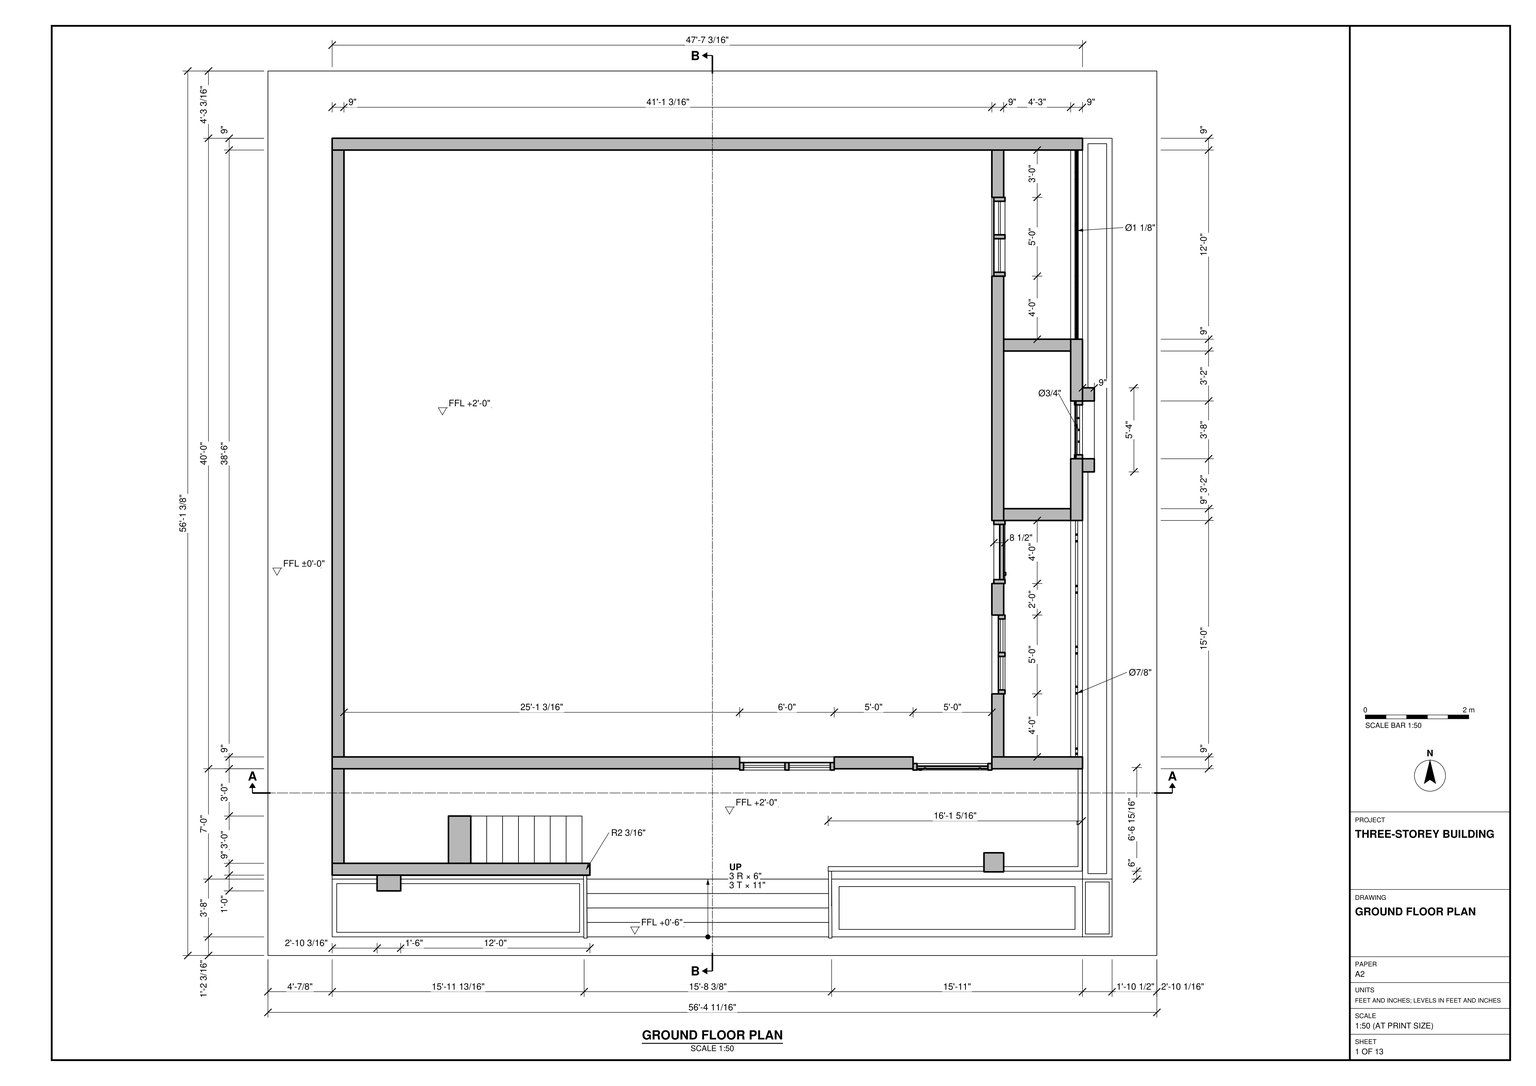
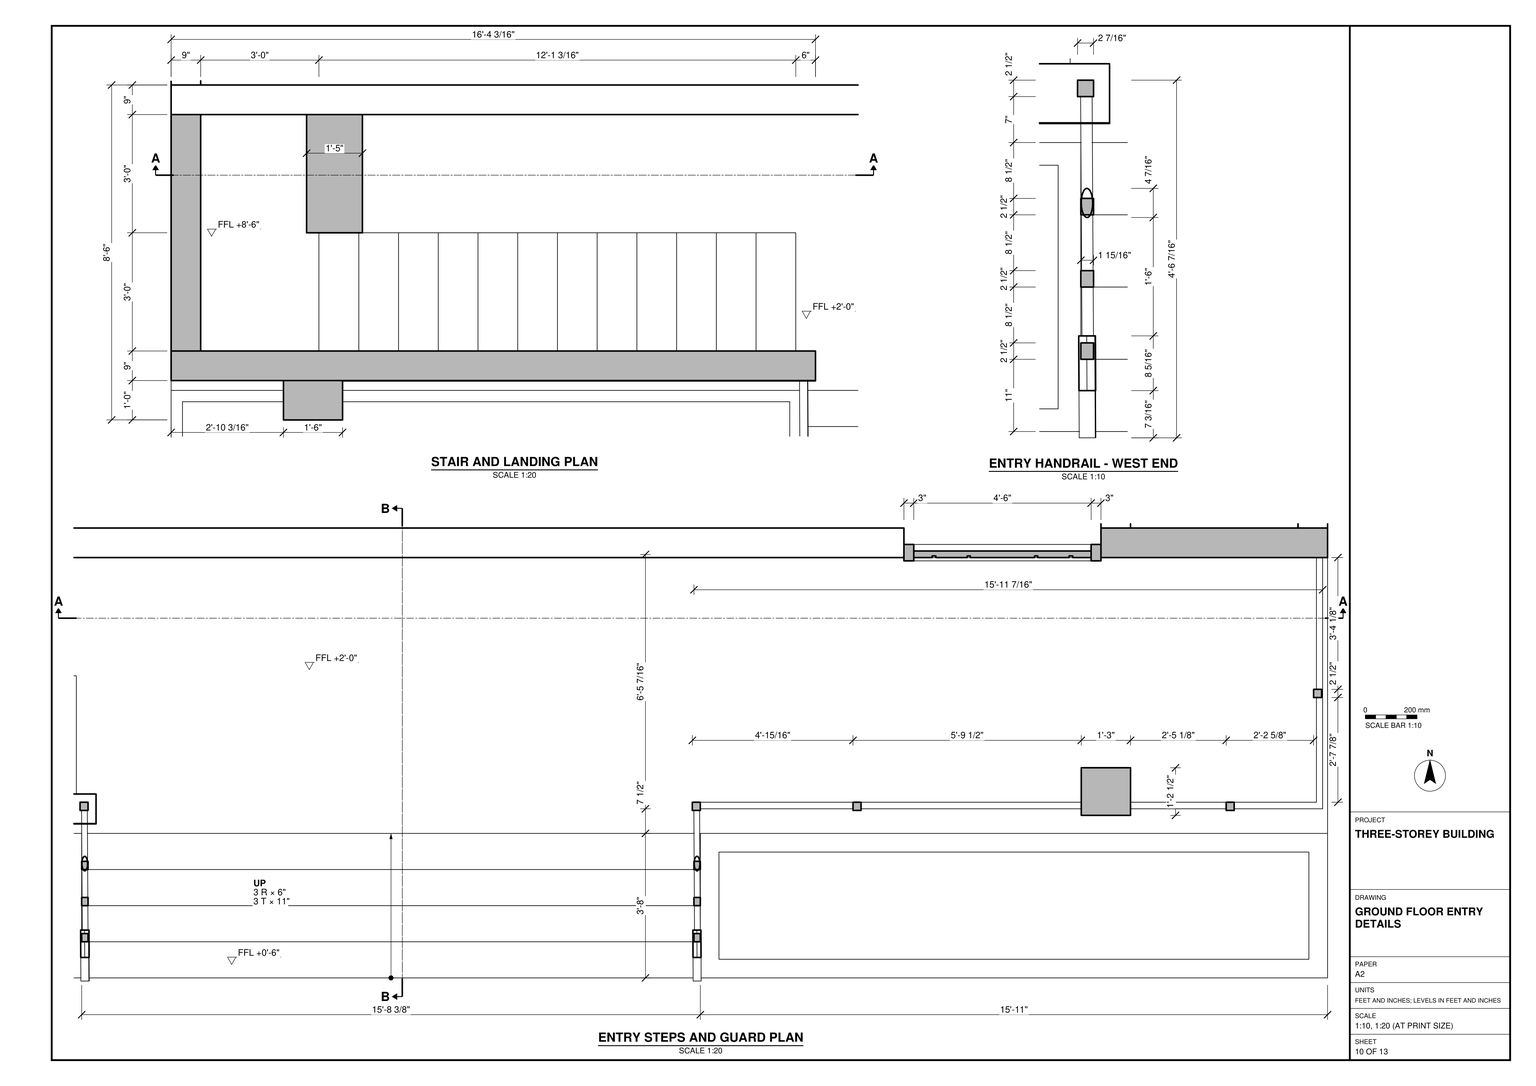
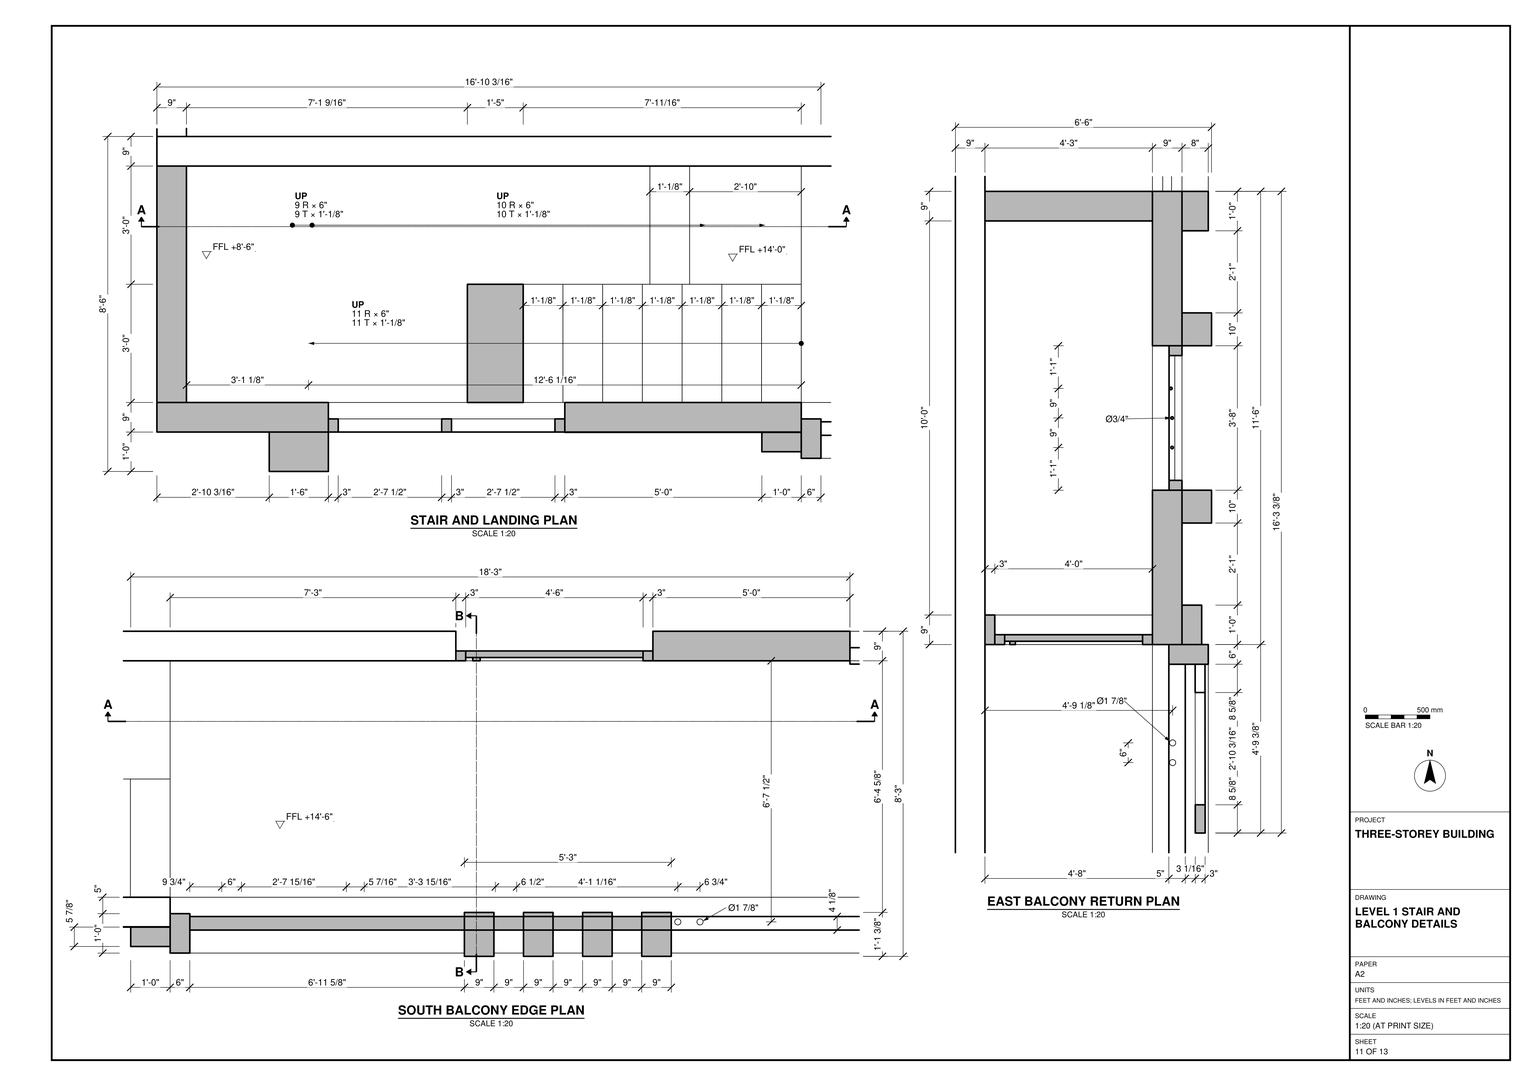
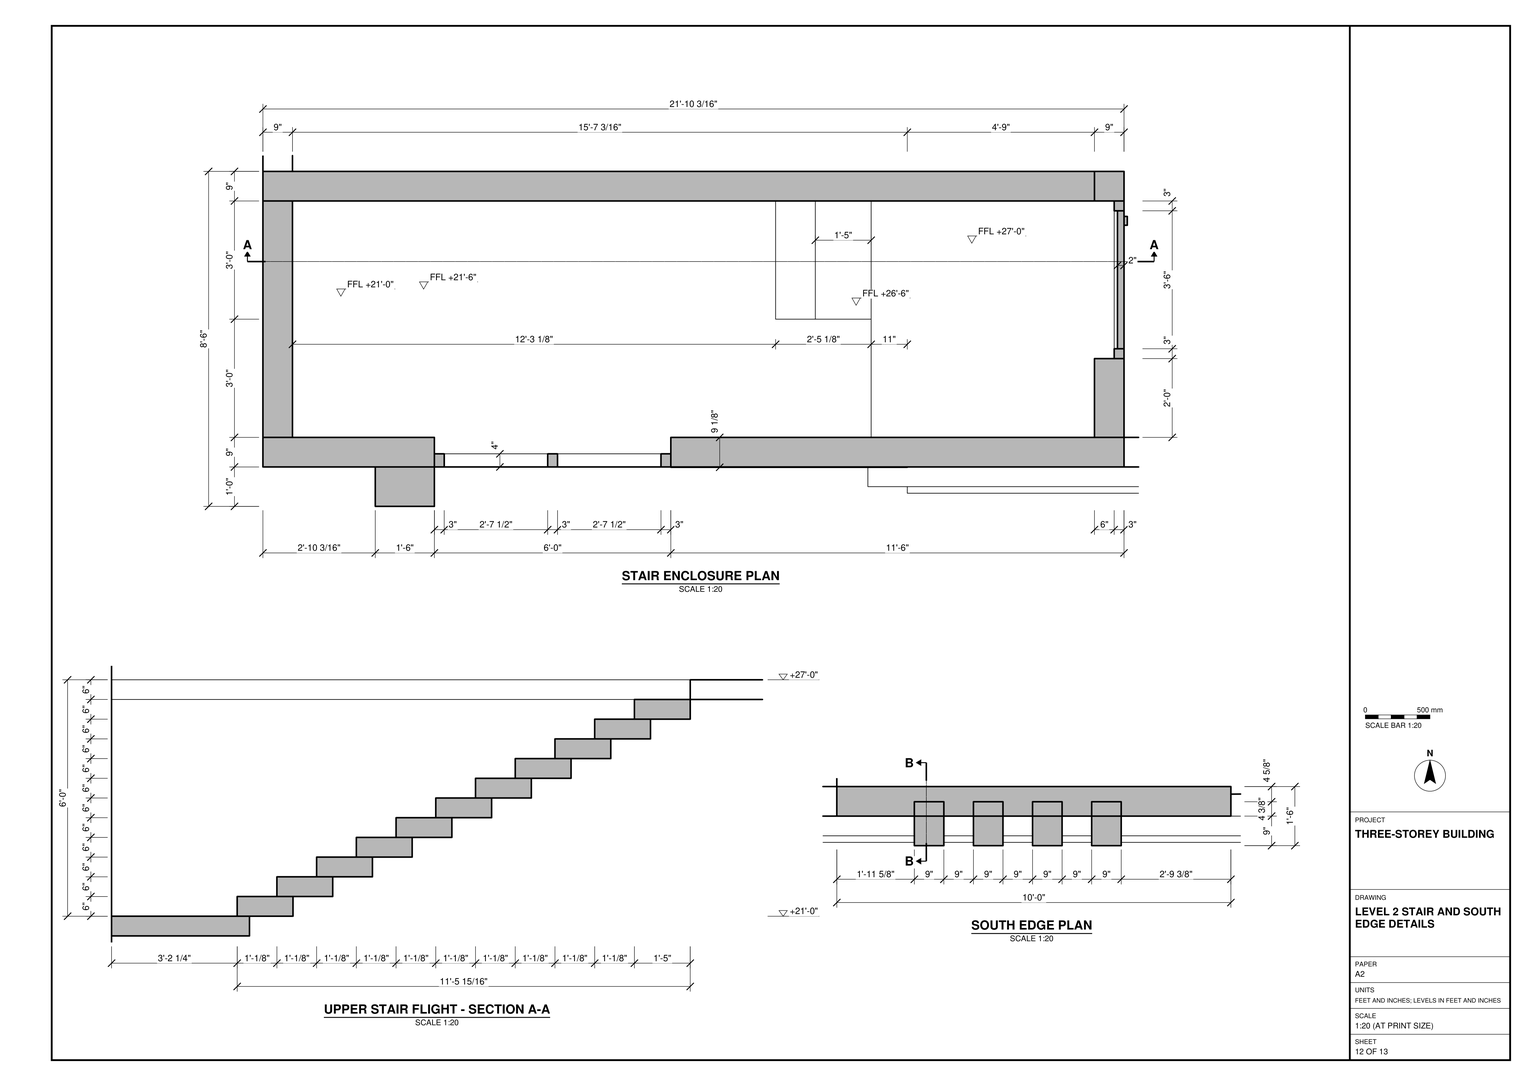
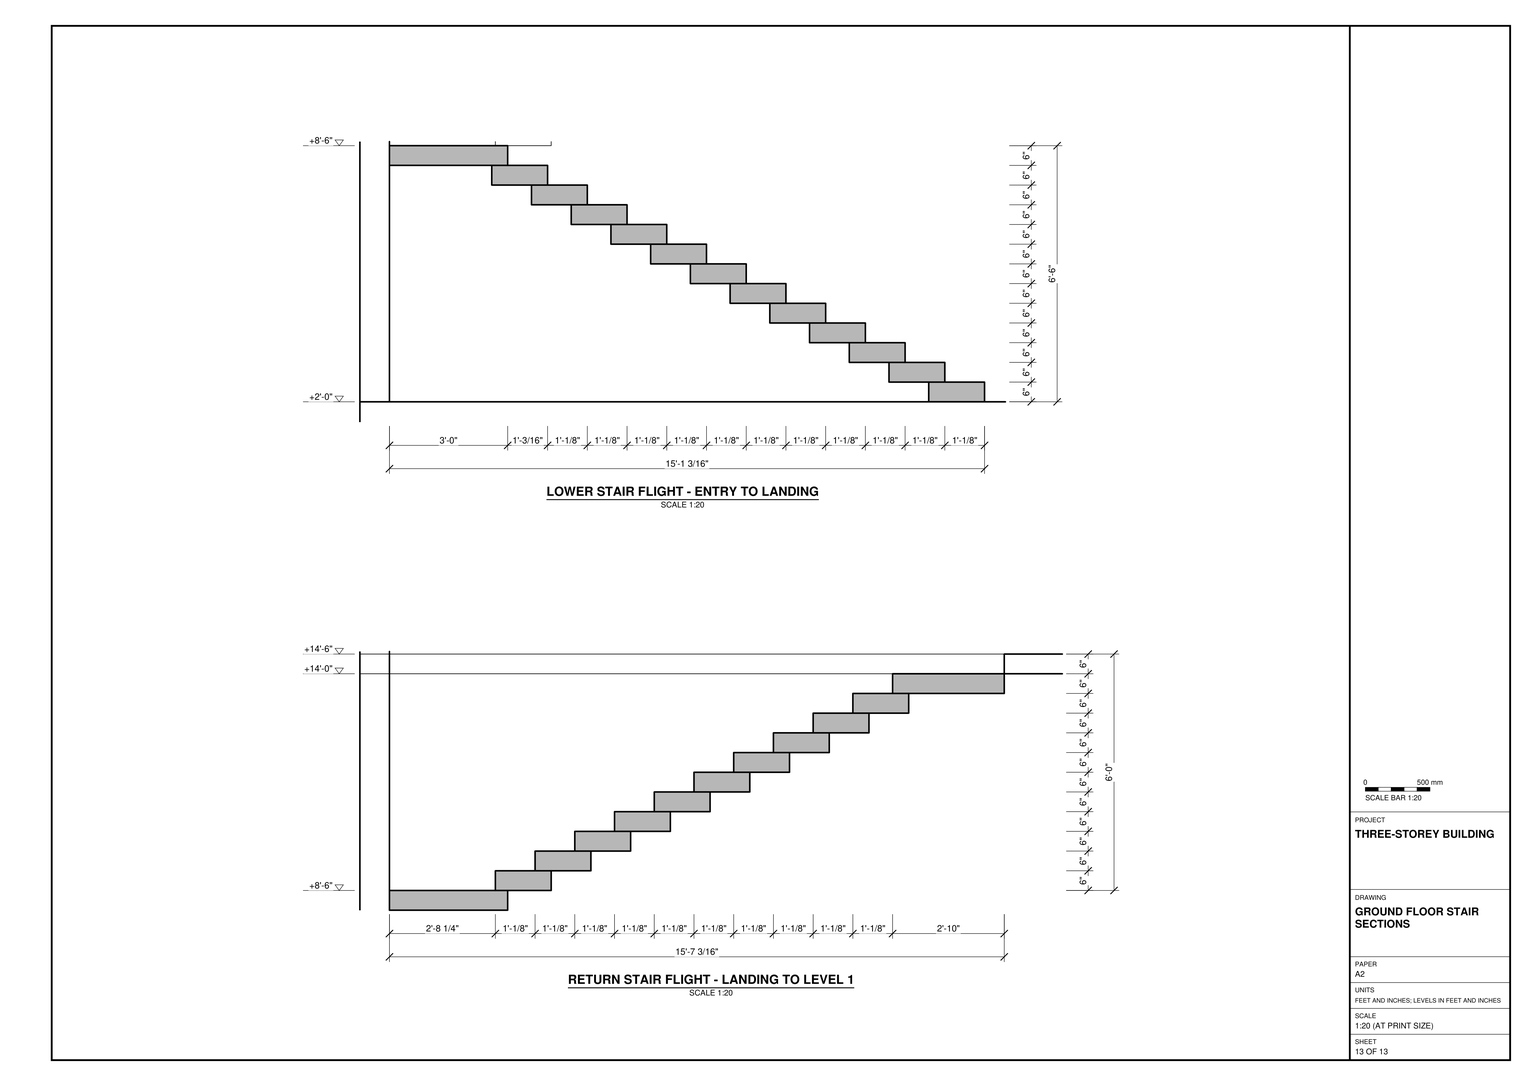
Build the three-storey building in SketchUp using task_files/diagram_01.pdf. Work in feet and inches. Orient the south entrance as shown on the plan. The overall model measures 56'-4 11/16" east to west, 56'-1 3/8" north to south and 43'-0" high. Use ±0'-0" as the ground datum and set the upper storey levels at +14'-6" and +27'-0". Distinguish the raised ground-floor surface at +2'-0" from the surrounding base.

Lay out the large open ground-floor space, the narrow bays along its east side and the entrance along its south side. Use the wall thicknesses shown, including the 9" walls, and place the door and window openings to match the plans. Model the broad entry steps and their handrails separately from the returning stair at the west end of the entrance. Align the stair flights, intermediate landings and slab openings so the stair connects the levels shown. Use the balcony details to shape the south edge and east return, including their guards. Complete the upper walls, floor slabs and roof to match the sheets.

Keep walls, slabs, roof and any furniture or built-in joinery shown as separate groups or components, and use components for repeated parts. Decor and loose items may be any suitable library components. Save one SketchUp model as output_files/three_storey_building_with_a_raised_entry_and_balconies.skp.

# SketchUp Ruby script. Lengths in inches.
U = 1.inch
M = Sketchup.active_model
def pt(a) = Geom::Point3d.new(a.map { |v| v * U })
def face(e, loops, mat)
  f = e.add_face(loops[0].map { |a| pt(a) })
  loops[1..].each { |l| e.add_face(l.map { |a| pt(a) }).erase! }
  f.material = f.back_material = mat if mat
  f
end
# faces: each face lists its corners as indices into pts; further lists are holes
def faces(e, pts, list, mat = nil) = list.each { |f| face(e, (f[0].is_a?(Array) ? f : [f]).map { |l| l.map { |i| pts[i] } }, mat) }
# xy, xz, yz: faces in a plane at the given z, y or x. An outline is a flat list of corners, or four numbers for a rectangle; further outlines are holes
def ring(l) = l.size == 4 ? [[l[0], l[1]], [l[2], l[1]], [l[2], l[3]], [l[0], l[3]]] : l.each_slice(2).to_a
def flat(e, list, mat, &to3) = list.each { |f| face(e, (f[0].is_a?(Array) ? f : [f]).map { |l| ring(l).map { |u, v| to3.(u, v) } }, mat) }
def xy(e, z, list, mat = nil) = flat(e, list, mat) { |x, y| [x, y, z] }
def xz(e, y, list, mat = nil) = flat(e, list, mat) { |x, z| [x, y, z] }
def yz(e, x, list, mat = nil) = flat(e, list, mat) { |y, z| [x, y, z] }
def lines(e, pts, list) = list.each { |a, b| e.add_line(pt(pts[a]), pt(pts[b])) }
# prism: a flat outline (further loops are holes) pulled along v
def prism(e, loops, v, mat = nil)
  f = face(e, loops, mat); d = Geom::Vector3d.new(v.map { |x| x * U })
  f.pushpull(f.normal.samedirection?(d) ? d.length : -d.length)
end
def box(e, o, s, mat = nil) = prism(e, [[o, [o[0] + s[0], o[1], o[2]], [o[0] + s[0], o[1] + s[1], o[2]], [o[0], o[1] + s[1], o[2]]]], [0, 0, s[2]], mat)
def at(x, y, z, deg = 0) = Geom::Transformation.translation(pt([x, y, z])) * Geom::Transformation.rotation(ORIGIN, Z_AXIS, deg.degrees)
def axes(o, x, y, z) = Geom::Transformation.new([*x, 0, *y, 0, *z, 0, *pt(o).to_a, 1])
def part(name) = M.definitions.add(name)
# library, detail: a bought-in or finely detailed component or shape, given as its bounding box
def library(name, o, s) = part(name).tap { |d| box(d.entities, o, s) }
def detail(e, o, s) = box(e.add_group.entities, o, s)
def put(e, d, t, mat = nil) = e.add_instance(d, t).tap { |i| i.material = mat if mat }
def group(e, t, mat = nil) = e.add_group.tap { |g| g.transformation = t; g.material = mat if mat }.entities
root = M.entities
M.materials.add("[Aluminum]").color = [179, 179, 179]
M.materials.add("[Color M01]").color = [226, 226, 226]
M.materials.add("[Color M02]").color = [198, 198, 198]
M.materials.add("[Color M03]").color = [170, 170, 170]
M.materials.add("[Color M06]").color = [86, 86, 86]
M.materials.add("[Color M09]").color = [0, 0, 0]
M.materials.add("[Grass Dark Green]").color = [106, 157, 55]
M.materials.add("[Metal Aluminum Anodized]").color = [202, 209, 219]
M.materials.add("[Metal Silver]").color = [234, 233, 238]
M.materials.add("[Translucent Glass Blue]").color = [100, 149, 237]
M.materials["[Translucent Glass Blue]"].alpha = 0.5
M.materials.add("[Translucent Glass Gray]").color = [128, 128, 128]
M.materials["[Translucent Glass Gray]"].alpha = 0.5
M.materials.add("[Wood Bamboo]").color = [177, 105, 43]
c1 = library("Group\#10",[0,0,0],[1.375,93,1.375])
c2 = library("Group\#22",[0,0,0],[2,54,2])
c3 = part("Group\#67")
box(c3.entities,[-6,0,0],[17,36,6])
c4 = part("Group\#17")
put(c4.entities,c3,at(102.77,0,18))
put(c4.entities,c3,at(139.05,0,0))
put(c4.entities,c3,at(30.19,0,54))
put(c4.entities,c3,at(78.58,0,30))
put(c4.entities,c3,at(42.29,0,48))
put(c4.entities,c3,at(18.1,0,60))
put(c4.entities,c3,at(90.67,0,24))
put(c4.entities,c3,at(126.96,0,6))
put(c4.entities,c3,at(66.48,0,36))
put(c4.entities,c3,at(54.38,0,42))
put(c4.entities,c3,at(114.86,0,12))
put(c4.entities,c3,at(6,0,66))
c5 = library("Group\#30",[0,0,0],[66,1.5,1.5])
c6 = library("Group\#33",[0,0,0],[54,2,102])
c7 = library("Group\#43",[0,0,0],[1,54,1])
c8 = library("Group\#16",[0,0,0],[1.625,38,69])
c9 = library("Group\#142",[0,0,0],[1.625,38,69])
c10 = library("Group\#51",[0,0,0],[66,2,2])
c11 = part("Group\#60")
box(c11.entities,[0,0,0],[4,2.91,144])
c12 = library("Group\#63",[0,0,0],[1.625,144,1.625])
c13 = library("Group\#64",[0,0,0],[0.75,0.75,30.1875])
c14 = part("Group\#72")
prism(c14.entities,[[[0,0,0],[0,3.125,0],[365,3.125,0],[365,264,0],[370,264,0],[370,0,0]]],[0,0,1.75])
c15 = library("Group\#73",[0,0,0],[1.875,1.875,35])
c16 = library("Group\#77",[0,0,0],[1.75,180,1.75])
c17 = library("Group\#78",[0,0,0],[0.875,0.875,22.1875])
c18 = library("Group\#80",[0,0,0],[2.625,144,2.625])
c19 = library("Group\#81",[0,0,0],[1.125,1.125,21.4375])
c20 = library("Group\#86",[0,0,0],[72,4,264])
c21 = part("Group\#118")
prism(c21.entities,[[[0,0,0],[0,5.25,0],[142.22,5.25,0],[142.22,83.66,0],[0,83.66,0],[0,88.35,0],[147.34,88.35,0],[147.34,0,0]]],[0,0,1.8125])
c22 = library("Group\#119",[0,0,0],[1.875,1.875,16.1875])
c23 = part("Group\#122")
prism(c23.entities,[[[0,0.5,0],[0,2.5,0],[189.55,2.5,0],[189.55,77.9375,0],[191.4375,77.9375,0],[191.4375,0.5,0]]],[0,0,3])
c24 = part("Group\#121")
box(c24.entities,[-0.5,0,0],[2.4375,2.5,36])
c25 = library("Group\#144",[0,0,0],[2.7,54.46,57])
c26 = library("Group\#130",[0,0,0],[2.8,54.46,57])
c27 = library("Group\#140",[0,0,0],[0.625,41,0.625])
c28 = library("Group\#141",[0,0,0],[0.875,41,0.875])
xz(root,61.08,[[240.23,64.88,242.67,67.88]])
xz(root,142.18,[[616.7,34,618.59,37],[616.7,42,618.59,45],[616.7,50,618.59,53],[616.7,58,618.59,61],[616.7,66,619.79,69]])
yz(root,560.09,[[65.68,42,67.68,45],[65.68,50,67.68,53],[65.68,58,67.68,61],[64.18,66,67.68,69]])
# 98 loose lines left out
g1 = group(root,at(-686.5,0,0))
box(g1,[686.5,0,0],[676.6875,673.375,6])
g2 = group(root,at(-303.91,142.18,6),"[Color M01]")
box(g2,[352.79,-84,0],[571.21,564,24])
g3 = group(root,at(-303.91,613.18,30),"[Color M01]")
box(g3,[352.79,0,0],[571.21,9,144])
g4 = group(root,at(551.09,142.18,30),"[Color M02]")
prism(g4,[[[0,141,0],[0,9,0],[0,9,144],[0,471,144],[0,471,0],[0,189,0],[0,189,108],[0,141,108]],[[0,375,36],[0,435,36],[0,435,108],[0,375,108]],[[0,57,36],[0,117,36],[0,117,108],[0,57,108]]],[9,0,0])
g5 = group(root,at(-303.91,142.18,30),"[Color M02]")
prism(g5,[[[795,9,0],[352.79,9,0],[352.79,9,144],[924,9,144],[924,9,0],[855,9,0],[855,9,108],[795,9,108]],[[663,9,108],[663,9,36],[735,9,36],[735,9,108]]],[0,-9,0])
g6 = group(root,at(611.09,331.18,30),"[Color M02]")
prism(g6,[[[0,138,0],[0,0,0],[0,0,360],[0,291,360],[0,291,294],[0,138,294]],[[0,91,36],[0,91,108],[0,47,108],[0,47,36]],[[0,91,258],[0,47,258],[0,47,186],[0,91,186]]],[9,0,0])
g7 = group(root,at(560.09,331.18,30),"[Color M01]")
prism(g7,[[[51,9,0],[0,9,0],[0,9,294],[51,9,294],[51,9,258],[3,9,258],[3,9,150],[51,9,150]]],[0,-9,0])
g8 = group(root,at(560.09,460.18,30),"[Color M02]")
box(g8,[0,0,0],[51,9,294])
g9 = group(root,at(552.59,517.18,66),"[Color M09]")
xy(g9,0,[[0,0,8.5,60]])
xy(g9,3,[[0,3,8.5,28.5],[0,31.5,8.5,57]])
xy(g9,69,[[0,3,8.5,28.5],[0,31.5,8.5,57]])
xy(g9,72,[[0,0,8.5,28.5],[0,28.5,8.5,31.5],[0,31.5,8.5,60]])
xz(g9,0,[[0,0,8.5,72]])
xz(g9,3,[[0,3,8.5,69]])
xz(g9,28.5,[[0,3,8.5,69],[0,69,3,72],[3,69,7.5,72],[7.5,69,8.5,72]])
xz(g9,31.5,[[0,3,8.5,69],[0,69,3,72],[3,69,7.5,72],[7.5,69,8.5,72]])
xz(g9,57,[[0,3,8.5,69]])
xz(g9,60,[[0,0,8.5,72]])
yz(g9,8.5,[[0,0,60,0,60,72,31.5,72,31.5,69,57,69,57,3,31.5,3,31.5,72,28.5,72,28.5,3,3,3,3,69,28.5,69,28.5,72,0,72]])
put(root,c1,at(556.15,520.18,130.98),"[Color M09]")
put(root,c1,at(556.15,520.18,123.98),"[Color M09]")
put(root,c1,at(556.15,520.18,116.98),"[Color M09]")
put(root,c1,at(556.15,520.18,109.98),"[Color M09]")
put(root,c1,at(556.15,520.18,102.98),"[Color M09]")
put(root,c1,at(556.15,520.18,95.98),"[Color M09]")
put(root,c1,at(556.15,520.18,88.98),"[Color M09]")
put(root,c1,at(556.15,520.18,81.98),"[Color M09]")
put(root,c1,at(556.15,520.18,74.98),"[Color M09]")
put(root,c1,at(556.15,520.18,60.98))
g10 = group(root,at(552.59,283.18,30),"[Wood Bamboo]")
prism(g10,[[[0,48,0],[0,0,0],[0,0,108],[0,48,108]],[[0,45,3],[0,45,105],[0,3,105],[0,3,3]]],[8.5,0,0])
g11 = group(root,at(557.09,286.18,33),"[Wood Bamboo]")
prism(g11,[[[0,42,0],[0,42,102],[3,42,102],[3,42,79.3],[2.5,42,79.3],[2.5,42,78],[3,42,78],[3,42,51.6],[2.5,42,51.6],[2.5,42,50.4],[3,42,50.4],[3,42,30.3],[2.5,42,30.3],[2.5,42,29],[3,42,29],[3,42,0]]],[0,-42,0])
g12 = group(root,at(556.09,199.18,66),"[Color M09]")
prism(g12,[[[0,0,72],[0,60,72],[0,60,0],[0,0,0]],[[0,31.5,69],[0,31.5,3],[0,57,3],[0,57,69]],[[0,28.5,69],[0,3,69],[0,3,3],[0,28.5,3]]],[5,0,0])
g13 = group(root,at(552.59,517.18,66),"[Translucent Glass Blue]")
yz(g13,0,[[0,0,60,72]])
put(root,c2,at(557.59,202.18,130.56),"[Color M09]")
put(root,c2,at(557.59,202.18,123.56),"[Color M09]")
put(root,c2,at(557.59,202.18,116.56),"[Color M09]")
put(root,c2,at(557.59,202.18,109.56),"[Color M09]")
put(root,c2,at(557.59,202.18,102.56),"[Color M09]")
put(root,c2,at(557.59,202.18,95.56),"[Color M09]")
put(root,c2,at(557.59,202.18,88.56),"[Color M09]")
put(root,c2,at(557.59,202.18,81.56),"[Color M09]")
put(root,c2,at(557.59,202.18,74.56),"[Color M09]")
g14 = group(root,at(556.09,202.18,69),"[Translucent Glass Blue]")
yz(g14,0,[[0,0,54,66]])
g15 = group(root,at(560.09,289.54,71),"[Metal Aluminum Anodized]")
box(g15,[0,0,0],[1.5,2.0625,26.6875])
g16 = group(root,at(57.88,70.18,30))
g17 = group(g16,at(164.21,72,138,-180))
box(g17,[-23,0,0],[34,36,6])
put(g16,c3,at(140.02,72,126,-180))
put(g16,c3,at(103.73,72,108,-180))
put(g16,c3,at(67.44,72,90,-180))
put(g16,c4,at(31.16,0,0))
put(g16,c3,at(115.83,72,114,-180))
put(g16,c3,at(79.54,72,96,-180))
put(g16,c3,at(43.25,72,78,-180))
put(g16,c3,at(152.11,72,132,-180))
g18 = group(g16,at(0,0,72))
box(g18,[0,0,0],[36,72,6])
put(g16,c3,at(127.92,72,120,-180))
put(g16,c3,at(55.35,72,84,-180))
put(g16,c3,at(91.63,72,102,-180))
g19 = group(root,at(63.88,70.18,180))
put(g19,c3,at(164.21,72,138,-180))
put(g19,c3,at(140.02,72,126,-180))
put(g19,c3,at(103.73,72,108,-180))
put(g19,c3,at(67.44,72,90,-180))
put(g19,c4,at(31.16,0,0))
put(g19,c3,at(115.83,72,114,-180))
put(g19,c3,at(79.54,72,96,-180))
put(g19,c3,at(43.25,72,78,-180))
put(g19,c3,at(152.11,72,132,-180))
g20 = group(g19,at(0,0,72))
box(g20,[-6,0,0],[42,72,6])
put(g19,c3,at(127.92,72,120,-180))
put(g19,c3,at(55.35,72,84,-180))
put(g19,c3,at(91.63,72,102,-180))
g21 = group(root,at(48.88,61.18,30),"[Color M02]")
prism(g21,[[[0,9,468],[262.21,9,468],[262.21,9,300],[196.21,9,300],[196.21,9,0],[0,9,0]],[[124.21,9,420],[52.21,9,420],[52.21,9,156],[124.21,9,156]]],[0,-9,0])
g22 = group(root,at(48.88,70.18,30),"[Color M01]")
box(g22,[0,0,0],[9,72,468])
g23 = group(root,at(359.09,143.87,66),"[Color M09]")
prism(g23,[[[0,-2.6875,72],[0,-2.6875,0],[72,-2.6875,0],[72,-2.6875,72]],[[34.5,-2.6875,69],[34.5,-2.6875,3],[3,-2.6875,3],[3,-2.6875,69]],[[37.5,-2.6875,69],[69,-2.6875,69],[69,-2.6875,3],[37.5,-2.6875,3]]],[0,5.6875,0])
put(root,c5,at(362.09,143.28,130.17),"[Aluminum]")
put(root,c5,at(362.09,143.28,123.17),"[Aluminum]")
put(root,c5,at(362.09,143.28,116.17),"[Aluminum]")
put(root,c5,at(362.09,143.28,109.17),"[Aluminum]")
put(root,c5,at(362.09,143.28,102.17),"[Aluminum]")
put(root,c5,at(362.09,143.28,95.17),"[Aluminum]")
put(root,c5,at(362.09,143.28,88.17),"[Aluminum]")
put(root,c5,at(362.09,143.28,81.17),"[Aluminum]")
put(root,c5,at(362.09,143.28,74.17),"[Aluminum]")
put(root,c5,at(362.09,143.28,67.17))
g24 = group(root,at(362.09,146.87,69),"[Translucent Glass Blue]")
xz(g24,0,[[0,0,66,66]])
g25 = group(root,at(491.09,143.18,30),"[Wood Bamboo]")
prism(g25,[[[0,-2,0],[60,-2,0],[60,-2,108],[0,-2,108]],[[3,-2,105],[57,-2,105],[57,-2,3],[3,-2,3]]],[0,5,0])
put(root,c6,at(494.09,142.18,33),"[Wood Bamboo]")
g26 = group(root,at(495.69,141.18,72),"[Metal Aluminum Anodized]")
box(g26,[0,0,0],[1.9,1,24])
g27 = group(root,at(48.88,142.18,174))
prism(g27,[[[196.21,0,0],[0,0,0],[0,480,0],[571.21,480,0],[571.21,327,0],[511.21,327,0],[511.21,189,0],[571.21,189,0],[571.21,-81,0],[196.21,-81,0]]],[0,0,6])
g28 = group(root,at(551.09,142.18,180),"[Color M02]")
prism(g28,[[[0,480,0],[0,9,0],[0,9,144],[0,480,144]],[[0,435,108],[0,375,108],[0,375,36],[0,435,36]]],[9,0,0])
g29 = group(root,at(48.88,142.18,180),"[Color M02]")
prism(g29,[[[283.21,9,0],[0,9,0],[0,9,144],[511.21,9,144],[511.21,9,0],[343.21,9,0],[343.21,9,108],[283.21,9,108]],[[403.21,9,108],[403.21,9,36],[475.21,9,36],[475.21,9,108]]],[0,-9,0])
g30 = group(root,at(48.88,613.18,180),"[Color M01]")
box(g30,[0,0,0],[502.21,9,144])
g31 = group(root,at(48.88,151.18,30),"[Color M01]")
box(g31,[0,0,0],[9,462,144])
g32 = group(root,at(560.09,340.18,174))
box(g32,[0,0,0],[51,120,6])
g33 = group(root,at(556.09,517.18,216),"[Color M09]")
prism(g33,[[[5,60,0],[5,60,72],[5,0,72],[5,0,0]],[[5,31.5,3],[5,31.5,69],[5,57,69],[5,57,3]],[[5,3,69],[5,28.5,69],[5,28.5,3],[5,3,3]]],[-5,0,0])
put(root,c7,at(558.09,520.18,281.77),"[Color M09]")
put(root,c7,at(558.09,520.18,274.77),"[Color M09]")
put(root,c7,at(558.09,520.18,267.77),"[Color M09]")
put(root,c7,at(558.09,520.18,260.77),"[Color M09]")
put(root,c7,at(558.09,520.18,253.77),"[Color M09]")
put(root,c7,at(558.09,520.18,246.77),"[Color M09]")
put(root,c7,at(558.09,520.18,239.77),"[Color M09]")
put(root,c7,at(558.09,520.18,232.77),"[Color M09]")
put(root,c7,at(558.09,520.18,225.77),"[Color M09]")
g34 = group(root,at(556.09,520.18,219),"[Translucent Glass Blue]")
yz(g34,0,[[0,0,54,66]])
g35 = group(root,at(616.15,378.18,216),"[Aluminum]")
prism(g35,[[[0,0,0],[0,0,72],[0,44,72],[0,44,0]],[[0,3,3],[0,41,3],[0,41,69],[0,3,69]]],[3.9375,0,0])
g36 = group(root,at(614.09,378.18,66),"[Color M09]")
prism(g36,[[[6,0,0],[6,44,0],[6,44,72],[6,0,72]],[[6,3,69],[6,41,69],[6,41,3],[6,3,3]]],[-6,0,0])
put(root,c8,at(616.28,381.18,69),"[Color M09]")
put(root,c9,at(616.28,381.18,219),"[Color M09]")
g37 = group(root,at(616.15,381.18,219),"[Translucent Glass Gray]")
yz(g37,0,[[0,0,38,66]])
g38 = group(root,at(563.09,331.18,180),"[Wood Bamboo]")
prism(g38,[[[0,3,0],[0,3,108],[48,3,108],[48,3,0]],[[3,3,105],[3,3,3],[45,3,3],[45,3,105]]],[0,-3,0])
g39 = group(root,at(566.09,330.18,183),"[Wood Bamboo]")
box(g39,[0,2,0],[42,2,102])
g40 = group(root,at(567.67,331.18,217.86),"[Metal Aluminum Anodized]")
box(g40,[0,0,0],[1.6875,1,21.75])
g41 = group(root,at(452.09,142.18,216),"[Color M09]")
prism(g41,[[[0,-1,72],[0,-1,0],[72,-1,0],[72,-1,72]],[[34.5,-1,69],[34.5,-1,3],[3,-1,3],[3,-1,69]],[[37.5,-1,69],[69,-1,69],[69,-1,3],[37.5,-1,3]]],[0,5,0])
put(root,c10,at(455.09,142.68,280.2),"[Aluminum]")
put(root,c10,at(455.09,142.68,273.2),"[Aluminum]")
put(root,c10,at(455.09,142.68,266.2),"[Aluminum]")
put(root,c10,at(455.09,142.68,259.2),"[Aluminum]")
put(root,c10,at(455.09,142.68,252.2),"[Aluminum]")
put(root,c10,at(455.09,142.68,245.2),"[Aluminum]")
put(root,c10,at(455.09,142.68,238.2),"[Aluminum]")
put(root,c10,at(455.09,142.68,231.2),"[Aluminum]")
put(root,c10,at(455.09,142.68,224.2),"[Aluminum]")
g42 = group(root,at(455.09,146.18,219),"[Translucent Glass Blue]")
xz(g42,0,[[0,0,66,66]])
g43 = group(root,at(332.09,142.18,180),"[Wood Bamboo]")
prism(g43,[[[60,0,108],[0,0,108],[0,0,0],[60,0,0]],[[57,0,3],[3,0,3],[3,0,105],[57,0,105]]],[0,3,0])
g44 = group(root,at(335.09,143.18,183),"[Wood Bamboo]")
box(g44,[0,0,0],[54,2,102])
g45 = group(root,at(337.24,142.18,213.58),"[Metal Aluminum Anodized]")
box(g45,[0,0,0],[2.25,1,25.3125])
g46 = group(root,at(560.09,613.18,180),"[Color M01]")
box(g46,[0,0,0],[60,9,144])
g47 = group(root,at(48.88,151.18,324))
prism(g47,[[[0,-9,0],[0,471,0],[562.21,471,0],[562.21,180,0],[571.21,180,0],[571.21,-90,0],[196.21,-90,0],[196.21,-81,0],[185.21,-81,0],[185.21,-9,0]]],[0,0,6])
g48 = group(root,at(620.09,451.18,162),"[Color M06]")
prism(g48,[[[8,6,0],[8,171,0],[8,171,180],[8,6,180]],[[8,18,18],[8,18,162],[8,162,162],[8,162,18]]],[-8,0,0])
g49 = group(root,at(611.09,469.18,180))
box(g49,[0,0,0],[9,144,12])
g50 = group(root,at(620.09,584.6,180),"[Metal Aluminum Anodized]")
put(g50,c11,at(0,10,0))
put(g50,c11,at(0,5,0))
put(g50,c11,at(0,15,0))
put(g50,c11,at(0,0,0))
put(g50,c11,at(0,20,0))
put(g50,c11,at(0,25,0))
g51 = group(root,at(614.22,469.18,222))
box(g51,[0,0,0],[2.6875,144,2.25])
put(root,c12,at(614.75,469.18,218.29))
put(root,c12,at(614.75,469.18,213.29))
put(root,c12,at(614.75,469.18,208.29))
put(root,c12,at(614.75,469.18,203.29))
put(root,c12,at(614.75,469.18,198.29))
put(root,c12,at(614.75,469.18,193.29))
put(root,c12,at(614.75,469.18,188.29))
put(root,c13,at(615.19,482.66,192))
put(root,c13,at(615.19,487.41,192))
put(root,c13,at(615.19,522.6,192))
put(root,c13,at(615.19,526.98,192))
put(root,c13,at(615.19,582.1,192))
put(root,c13,at(615.19,587.23,192))
put(root,c13,at(615.19,605.41,192))
put(root,c13,at(615.19,608.66,192))
put(root,c13,at(615.19,531.98,192))
put(root,c13,at(615.19,477.66,192))
put(root,c13,at(615.19,577.1,192))
g52 = group(root,at(620.09,372.18,60))
prism(g52,[[[9,-4,-4],[9,60,-4],[9,60,238],[9,-4,238]],[[9,6,228],[9,50,228],[9,50,6],[9,6,6]]],[-9,0,0])
g53 = group(root,at(245.09,57.18,180),"[Color M03]")
xy(g53,0,[[0,-4,0,8,371,8,371,274,383,274,383,-4]])
xy(g53,6,[[6,-4,383,-4,383,268,371,268,371,8,6,8]])
xy(g53,138,[[6,-4,6,8,371,8,371,268,383,268,383,-4]])
xy(g53,144,[[0,-4,383,-4,383,274,371,274,371,8,0,8]])
xz(g53,-4,[[0,0,383,0,383,6,6,6,6,138,383,138,383,144,0,144]])
xz(g53,8,[[0,0,0,144,371,144,371,138,6,138,6,6,371,6,371,0]])
xz(g53,268,[[371,6,383,138]])
xz(g53,274,[[371,0,383,144]])
yz(g53,0,[[-4,0,8,144]])
yz(g53,6,[[-4,6,8,138]])
yz(g53,371,[[8,0,8,6,268,6,268,138,8,138,8,144,274,144,274,0]])
yz(g53,383,[[-4,0,274,0,274,144,-4,144,-4,138,268,138,268,6,-4,6]])
g54 = group(root,at(233.09,55.18,168))
xy(g54,-6,[[0,0,0,6,387,6,387,288,393,288,393,0]])
xy(g54,12,[[12,0,393,0,393,276,387,276,387,6,12,6]])
xy(g54,156,[[12,0,12,6,387,6,387,276,393,276,393,0]])
xy(g54,175,[[0,0,393,0,393,288,387,288,387,6,0,6]])
xz(g54,0,[[0,-6,393,-6,393,12,12,12,12,156,393,156,393,175,0,175]])
xz(g54,6,[[0,-6,0,175,387,175,387,156,12,156,12,12,387,12,387,-6]])
xz(g54,276,[[387,12,393,156]])
xz(g54,288,[[387,-6,393,175]])
yz(g54,0,[[0,-6,6,175]])
yz(g54,12,[[0,12,6,156]])
yz(g54,387,[[6,-6,6,12,276,12,276,156,288,156,288,-6],[6,156,288,175]])
yz(g54,393,[[0,-6,288,-6,288,175,0,175,0,156,276,156,276,12,0,12]])
g55 = group(root,at(245.09,65.18,180))
prism(g55,[[[376,-5,0],[0,-5,0],[0,5,0],[366,5,0],[366,266,0],[376,266,0]]],[0,0,12])
g56 = group(root,at(251.09,57.18,311.2),"[Color M06]")
xy(g56,-2.2,[[0,0,0,8,365,8,365,268,373,268,373,0]])
xy(g56,6.8,[[0,0,373,0,373,268,365,268,365,8,0,8]])
xz(g56,0,[[0,-2.2,373,6.8]])
xz(g56,8,[[0,-2.2,365,6.8]])
xz(g56,268,[[365,-2.2,373,6.8]])
yz(g56,0,[[0,-2.2,8,6.8]])
yz(g56,365,[[8,-2.2,268,1.8],[8,1.8,268,6.8]])
yz(g56,373,[[0,-2.2,268,6.8]])
g57 = group(root,at(251.09,60.18,227))
prism(g57,[[[0,0,0],[0,4.125,0],[365,4.125,0],[365,265,0],[370,265,0],[370,0,0]]],[0,0,3.5625])
put(root,c14,at(251.09,61.18,218.96))
put(root,c14,at(251.09,61.18,212.96))
put(root,c14,at(251.09,61.18,206.96))
put(root,c14,at(251.09,61.18,200.96))
put(root,c14,at(251.09,61.18,194.96))
put(root,c15,at(259.875,61.74,192))
put(root,c15,at(265.875,61.74,192))
put(root,c15,at(297.81,61.74,192))
put(root,c15,at(303.24,61.74,192))
put(root,c15,at(343.18,61.74,192))
put(root,c15,at(349.68,61.74,192))
put(root,c15,at(398.74,61.74,192))
put(root,c15,at(405.49,61.74,192))
put(root,c15,at(455.68,61.74,192))
put(root,c15,at(462.99,61.74,192))
put(root,c15,at(497.43,61.74,192))
put(root,c15,at(503.43,61.74,192))
put(root,c15,at(537.12,61.74,192))
put(root,c15,at(543.12,61.74,192))
put(root,c15,at(579.74,61.74,192))
put(root,c15,at(585.74,61.74,192))
put(root,c15,at(616.31,61.74,192))
put(root,c15,at(616.31,86.68,192))
put(root,c15,at(610.31,61.74,192))
put(root,c15,at(616.31,92.68,192))
put(root,c15,at(616.31,133.37,192))
put(root,c15,at(616.31,139.37,192))
put(root,c15,at(616.31,173.18,192))
put(root,c15,at(616.31,179.18,192))
put(root,c15,at(616.31,229.56,192))
put(root,c15,at(616.31,235.56,192))
put(root,c15,at(616.31,294.31,192))
put(root,c15,at(616.31,300.31,192))
g58 = group(root,at(611.09,151.18,30),"[Color M06]")
box(g58,[0,0,0],[9,180,36])
g59 = group(root,at(611.09,469.18,30),"[Color M06]")
box(g59,[0,0,0],[9,144,36])
g60 = group(root,at(614.78,151.18,87.93))
box(g60,[0,0,0],[3.6875,180,2.125])
put(root,c16,at(614.72,151.18,83.4))
put(root,c16,at(614.72,151.18,78.4))
put(root,c16,at(614.72,151.18,73.4))
put(root,c16,at(614.72,151.18,68.4))
put(root,c17,at(615.15,153.16,66))
put(root,c17,at(615.15,157.04,66))
put(root,c17,at(615.15,199.16,66))
put(root,c17,at(615.15,204.16,66))
put(root,c17,at(615.15,229.6,66))
put(root,c17,at(615.15,234.6,66))
put(root,c17,at(615.15,275.85,66))
put(root,c17,at(615.15,280.85,66))
put(root,c17,at(615.15,314.97,66))
put(root,c17,at(615.15,319.97,66))
g61 = group(root,at(612.84,469.18,87.4375))
box(g61,[0,0,0],[5.125,144,2.5625])
put(root,c18,at(614.28,469.18,82.17))
put(root,c18,at(614.28,469.18,77.17))
put(root,c18,at(614.28,469.18,72.17))
put(root,c18,at(614.28,469.18,67.17))
put(root,c19,at(615.03,472.05,66))
put(root,c19,at(615.03,477.05,66))
put(root,c19,at(615.03,511.49,66))
put(root,c19,at(615.03,516.49,66))
put(root,c19,at(615.03,551.36,66))
put(root,c19,at(615.03,556.36,66))
put(root,c19,at(615.03,590.49,66))
put(root,c19,at(615.03,595.49,66))
g62 = group(root,at(624.09,285.78,186),"[Metal Silver]")
prism(g62,[[[3,39.4,0],[3,39.4,132],[3.05,-12,132],[3.05,-12,0]],[[3.01,30.8,123.39],[3.01,30.8,8.61],[3.04,-3.39,8.61],[3.04,-3.39,123.39]]],[-3,0,0])
g63 = group(root,at(627.1,282.39,194.61),"[Translucent Glass Gray]")
p = [[0.03,0,0],[0.03,0,114.79],[0,34.19,114.79],[0,34.19,0]]
faces(g63,p,[[0,1,2,3]])
g64 = group(root,at(545.09,58.18,30),"[Color M02]")
xy(g64,0,[[0,5.5,15,20]])
xy(g64,129,[[0,20,15,84]])
xy(g64,144,[[0,20,15,84]])
xy(g64,279,[[0,20,15,84]])
xy(g64,294,[[0,5.5,15,84]])
xz(g64,5.5,[[0,0,15,294]])
xz(g64,20,[[0,0,15,129],[0,144,15,279]])
xz(g64,84,[[0,129,15,144],[0,279,15,294]])
yz(g64,0,[[5.5,0,5.5,294,84,294,84,279,20,279,20,144,84,144,84,129,20,129,20,0]])
yz(g64,15,[[5.5,0,20,0,20,129,84,129,84,144,5.5,144],[5.5,144,20,144,20,279,84,279,84,294,5.5,294]])
# 1 loose lines left out
g65 = group(root,at(560.09,142.18,309),"[Color M02]")
box(g65,[0,0,0],[56,11.15,15])
put(root,c20,at(101.09,61.18,186),"[Color M09]")
g66 = group(root,at(138.59,61.18,189),"[Translucent Glass Blue]")
xz(g66,0,[[0,0,31.5,66]])
g67 = group(root,at(104.09,61.18,189),"[Translucent Glass Blue]")
xz(g67,0,[[0,0,31.5,66]])
g68 = group(root,at(138.59,61.18,258),"[Translucent Glass Blue]")
xz(g68,0,[[0,0,31.5,61]])
g69 = group(root,at(104.09,61.18,258),"[Translucent Glass Blue]")
xz(g69,0,[[0,0,31.5,61]])
g70 = group(root,at(138.59,61.18,386),"[Translucent Glass Blue]")
xz(g70,0,[[0,0,31.5,61]])
g71 = group(root,at(104.09,61.18,386),"[Translucent Glass Blue]")
xz(g71,0,[[0,0,31.5,61]])
g72 = group(root,at(104.09,61.18,322),"[Translucent Glass Blue]")
xz(g72,0,[[0,0,31.5,61]])
g73 = group(root,at(138.59,61.18,322),"[Translucent Glass Blue]")
xz(g73,0,[[0,0,31.5,61]])
g74 = group(root,at(83.09,49.18,30))
xy(g74,-24,[[0,0,18,12]])
xy(g74,420,[[[18,0,18,12,228,12,228,102,360,102,360,0],[240,24,252,90],[264,24,276,90],[288,24,300,90],[312,24,324,90],[336,24,348,90]]])
xy(g74,438,[[[0,0,360,0,360,102,228,102,228,12,0,12],[336,24,348,90],[312,24,324,90],[288,24,300,90],[264,24,276,90],[240,24,252,90]]])
xz(g74,0,[[0,-24,18,-24,18,420,360,420,360,438,0,438]])
xz(g74,12,[[0,-24,18,438],[18,420,228,438]])
xz(g74,24,[[240,420,252,438],[264,420,276,438],[288,420,300,438],[312,420,324,438],[336,420,348,438]],"[Color M09]")
xz(g74,90,[[240,420,252,438],[264,420,276,438],[288,420,300,438],[312,420,324,438],[336,420,348,438]],"[Color M09]")
xz(g74,102,[[228,420,360,438]])
yz(g74,0,[[0,-24,12,438]])
yz(g74,18,[[0,-24,12,420]])
yz(g74,228,[[12,420,102,438]])
yz(g74,240,[[24,420,90,438]],"[Color M09]")
yz(g74,252,[[24,420,90,438]],"[Color M09]")
yz(g74,264,[[24,420,90,438]],"[Color M09]")
yz(g74,276,[[24,420,90,438]],"[Color M09]")
yz(g74,288,[[24,420,90,438]],"[Color M09]")
yz(g74,300,[[24,420,90,438]],"[Color M09]")
yz(g74,312,[[24,420,90,438]],"[Color M09]")
yz(g74,324,[[24,420,90,438]],"[Color M09]")
yz(g74,336,[[24,420,90,438]],"[Color M09]")
yz(g74,348,[[24,420,90,438]],"[Color M09]")
yz(g74,360,[[0,420,102,438]])
g75 = group(root,at(48.88,142.18,330))
box(g75,[0,0,0],[253.21,9,168])
g76 = group(root,at(302.09,70.18,330),"[Color M02]")
prism(g76,[[[0,81,0],[0,72,0],[0,72,108],[0,24,108],[0,24,0],[0,0,0],[0,0,168],[0,81,168]]],[9,0,0])
g77 = group(root,at(308.09,94.18,330),"[Wood Bamboo]")
prism(g77,[[[0,0,108],[0,48,108],[0,48,0],[0,0,0]],[[0,45,105],[0,3,105],[0,3,3],[0,45,3]]],[3,0,0])
g78 = group(root,at(309.09,97.18,333),"[Wood Bamboo]")
box(g78,[0,0,0],[2,42,102])
g79 = group(root,at(57.88,70.18,450))
box(g79,[0,0,0],[244.21,72,6])
g80 = group(root,at(311.09,61.18,330),"[Color M06]")
box(g80,[0,0,0],[120,9,64])
g81 = group(root,at(334.69,52.18,186),"[Color M03]")
box(g81,[0,0,0],[8.99,13.375,214])
g82 = group(root,at(352.69,52.18,186),"[Color M03]")
box(g82,[0,0,0],[8.99,13.375,214])
g83 = group(root,at(370.69,52.18,186),"[Color M03]")
box(g83,[0,0,0],[8.99,13.375,214])
g84 = group(root,at(388.69,52.18,186),"[Color M03]")
box(g84,[0,0,0],[8.99,13.375,214])
g85 = group(root,at(611.09,67.87,330),"[Color M09]")
box(g85,[0,0,0],[2.625,2.3125,58])
g86 = group(root,at(611.09,67.87,330),"[Color M06]")
xy(g86,0,[[0,135.64,9,263.3125]])
xy(g86,11,[[8.5,135.64,9,263.3125]])
xy(g86,12,[[8.5,135.64,9,263.3125]])
xy(g86,18,[[8.5,135.64,9,263.3125]])
xy(g86,19,[[8.5,135.64,9,263.3125]])
xy(g86,25,[[8.5,135.64,9,263.3125]])
xy(g86,26,[[8.5,135.64,9,263.3125]])
xy(g86,32,[[8.5,135.64,9,263.3125]])
xy(g86,33,[[8.5,135.64,9,263.3125]])
xy(g86,39,[[8.5,135.64,9,263.3125]])
xy(g86,40,[[8.5,135.64,9,263.3125]])
xy(g86,46,[[8.5,135.64,9,263.3125]])
xy(g86,47,[[8.5,135.64,9,263.3125]])
xy(g86,53,[[8.5,135.64,9,263.3125]])
xy(g86,54,[[8.5,135.64,9,263.3125]])
xy(g86,58,[[-180,0,-180,2.3125,0,2.3125,0,135.64,2.625,135.64,2.625,0]])
xy(g86,60,[[0,135.64,9,263.3125]])
xy(g86,62.5,[[-180,0,2.625,0,2.625,135.64,0,135.64,0,2.3125,-180,2.3125]],"[Color M09]")
xz(g86,0,[[-180,58,2.625,62.5]],"[Color M09]")
xz(g86,2.3125,[[-180,58,0,62.5]],"[Color M09]")
xz(g86,135.64,[[0,0,9,0,9,11,8.5,11,8.5,12,9,12,9,18,8.5,18,8.5,19,9,19,9,25,8.5,25,8.5,26,9,26,9,32,8.5,32,8.5,33,9,33,9,39,8.5,39,8.5,40,9,40,9,46,8.5,46,8.5,47,9,47,9,53,8.5,53,8.5,54,9,54,9,60,2.625,60,2.625,58,0,58],[0,58,2.625,60],[0,60,2.625,62.5]])
xz(g86,263.3125,[[0,0,0,60,9,60,9,54,8.5,54,8.5,53,9,53,9,47,8.5,47,8.5,46,9,46,9,40,8.5,40,8.5,39,9,39,9,33,8.5,33,8.5,32,9,32,9,26,8.5,26,8.5,25,9,25,9,19,8.5,19,8.5,18,9,18,9,12,8.5,12,8.5,11,9,11,9,0]])
yz(g86,-180,[[0,58,2.3125,62.5]])
yz(g86,0,[[135.64,0,263.3125,60]])
yz(g86,0,[[2.3125,58,135.64,62.5]],"[Color M09]")
yz(g86,2.625,[[0,58,135.64,62.5]],"[Color M09]")
yz(g86,8.5,[[135.64,11,263.3125,12],[135.64,18,263.3125,19],[135.64,25,263.3125,26],[135.64,32,263.3125,33],[135.64,39,263.3125,40],
  [135.64,46,263.3125,47],[135.64,53,263.3125,54]])
yz(g86,9,[[135.64,0,263.3125,11],[135.64,12,263.3125,18],[135.64,19,263.3125,25],[135.64,26,263.3125,32],[135.64,33,263.3125,39],
  [135.64,40,263.3125,46],[135.64,47,263.3125,53],[135.64,54,263.3125,60]])
g87 = group(root,at(611.09,70.18,330),"[Translucent Glass Gray]")
p = [[2.625,0,0],[2.625,0,58],[0,133.32,58],[0,133.32,0]]
faces(g87,p,[[0,1,2,3]])
g88 = group(root,at(431.09,67.87,330),"[Translucent Glass Gray]")
p = [[0,0,0],[0,0,58],[180,2.3125,58],[180,2.3125,0]]
faces(g88,p,[[0,1,2,3]])
g89 = group(root,at(611.09,203.51,390))
box(g89,[0,0,0],[9,418.68,5])
g90 = group(root,at(443.09,68.9,455.97),"[Color M09]")
box(g90,[0,0,0],[2.5,6.375,5.375])
g91 = group(root,at(443.09,80.9,455.97),"[Color M09]")
box(g91,[0,0,0],[2.5,6.375,5.375])
g92 = group(root,at(443.09,92.9,455.97),"[Color M09]")
box(g92,[0,0,0],[2.5,6.375,5.375])
g93 = group(root,at(443.09,104.9,455.97),"[Color M09]")
box(g93,[0,0,0],[2.5,6.375,5.375])
g94 = group(root,at(443.09,116.9,455.97),"[Color M09]")
box(g94,[0,0,0],[2.5,6.375,5.375])
g95 = group(root,at(443.09,128.9,455.97),"[Color M09]")
box(g95,[0,0,0],[2.5,6.375,5.375])
g96 = group(root,at(48.88,61.18,498),"[Color M03]")
box(g96,[0,0,0],[113.05,90,18])
put(root,c21,at(161.93,62.83,514.1875))
put(root,c21,at(161.93,62.83,510.1875))
put(root,c21,at(161.93,62.83,506.1875))
put(root,c21,at(161.93,62.83,502.1875))
put(root,c22,at(167.64,64.92,498))
put(root,c22,at(172.64,64.92,498))
put(root,c22,at(208.64,64.92,498))
put(root,c22,at(213.64,64.92,498))
put(root,c22,at(249.64,64.92,498))
put(root,c22,at(254.64,64.92,498))
put(root,c22,at(290.64,64.92,498))
put(root,c22,at(295.64,64.92,498))
put(root,c22,at(305.52,72.11,498))
put(root,c22,at(305.52,77.11,498))
put(root,c22,at(305.52,137.8,498))
put(root,c22,at(305.52,142.8,498))
put(root,c22,at(300.02,147.67,498))
put(root,c22,at(295.02,147.67,498))
put(root,c22,at(271.02,147.67,498))
put(root,c22,at(266.02,147.67,498))
put(root,c22,at(230.02,147.67,498))
put(root,c22,at(225.02,147.67,498))
put(root,c22,at(189.02,147.67,498))
put(root,c22,at(184.02,147.67,498))
put(root,c22,at(305.52,112.92,498))
put(root,c22,at(305.52,107.92,498))
g97 = group(root,at(245.09,14.18,6))
prism(g97,[[[184,44,0],[184,44,24],[184,33,24],[184,33,18],[184,22,18],[184,22,12],[184,11,12],[184,11,6],[184,0,6],[184,0,0]]],[-188.375,0,0])
g98 = group(root,at(427.15,65.18,66))
prism(g98,[[[-0.6875,-1,0],[-0.6875,2.5,0],[189.55,2.5,0],[189.55,77.9375,0],[192.64,77.9375,0],[192.64,-1,0]]],[0,0,3])
put(root,c23,at(427.15,65.18,58))
put(root,c23,at(427.15,65.18,50))
put(root,c23,at(427.15,65.18,42))
put(root,c23,at(427.15,65.18,34))
put(root,c23,at(427.15,65.18,26))
put(root,c24,at(476.09,65.18,30))
put(root,c24,at(589.72,65.18,30))
put(root,c24,at(616.34,99.56,30))
put(root,c25,at(426.65,13.22,12))
put(root,c26,at(240.21,13.22,12))
g99 = group(root,at(48.88,151.18,180),"[Color M01]")
box(g99,[0,0,0],[9,462,144])
g100 = group(root,at(48.88,613.18,330))
box(g100,[0,0,0],[562.21,9,60])
g101 = group(root,at(48.88,151.18,330),"[Color M01]")
box(g101,[0,0,0],[9,462,60])
g102 = group(root,at(101.09,61.08,30),"[Color M06]")
prism(g102,[[[72,0,420],[72,0,156],[0,0,156],[0,0,0],[144,0,0],[144,0,420]]],[0,0.1,0])
g103 = group(root,at(615.09,378.18,66),"[Translucent Glass Gray]")
yz(g103,0,[[0,0,44,72]])
g104 = group(root,at(429.09,14.18,6))
xy(g104,0,[[0,0,191,44]])
xy(g104,6.3125,[[5.68,5.68,185.32,38.32]],"[Grass Dark Green]")
xy(g104,8,[[[0,0,191,44],[5.68,5.68,185.32,38.32]]])
xz(g104,0,[[0,0,191,8]])
xz(g104,5.68,[[5.68,6.3125,185.32,8]])
xz(g104,38.32,[[5.68,6.3125,185.32,8]])
xz(g104,44,[[0,0,191,8]])
yz(g104,0,[[0,0,44,8]])
yz(g104,5.68,[[5.68,6.3125,38.32,8]])
yz(g104,185.32,[[5.68,6.3125,38.32,8]])
yz(g104,191,[[0,0,44,8]])
g105 = group(root,at(620.09,58.18,6))
xy(g105,0,[[0,0,22.53,564]])
xy(g105,6.6875,[[4.14,4.14,18.39,559.86]],"[Grass Dark Green]")
xy(g105,8,[[[0,0,22.53,564],[4.14,4.14,18.39,559.86]]])
xz(g105,0,[[0,0,22.53,8]])
xz(g105,4.14,[[4.14,6.6875,18.39,8]])
xz(g105,559.86,[[4.14,6.6875,18.39,8]])
xz(g105,564,[[0,0,22.53,8]])
yz(g105,0,[[0,0,564,8]])
yz(g105,4.14,[[4.14,6.6875,559.86,8]])
yz(g105,18.39,[[4.14,6.6875,559.86,8]])
yz(g105,22.53,[[0,0,564,8]])
g106 = group(root,at(620.09,14.18,6))
xy(g106,0,[[0,0,22.53,44]])
xy(g106,7.5625,[[2.2,2.2,20.32,41.8]],"[Grass Dark Green]")
xy(g106,8,[[[0,0,22.53,44],[2.2,2.2,20.32,41.8]]])
xz(g106,0,[[0,0,22.53,8]])
xz(g106,2.2,[[2.2,7.5625,20.32,8]])
xz(g106,41.8,[[2.2,7.5625,20.32,8]])
xz(g106,44,[[0,0,22.53,8]])
yz(g106,0,[[0,0,44,8]])
yz(g106,2.2,[[2.2,7.5625,41.8,8]])
yz(g106,20.32,[[2.2,7.5625,41.8,8]])
yz(g106,22.53,[[0,0,44,8]])
g107 = group(root,at(48.88,14.18,6))
xy(g107,0,[[0,0,191.83,44]])
xy(g107,6.625,[[3.45,3.45,188.38,40.55]],"[Grass Dark Green]")
xy(g107,8,[[[0,0,191.83,44],[3.45,3.45,188.38,40.55]]])
xz(g107,0,[[0,0,191.83,8]])
xz(g107,3.45,[[3.45,6.625,188.38,8]])
xz(g107,40.55,[[3.45,6.625,188.38,8]])
xz(g107,44,[[0,0,191.83,8]])
yz(g107,0,[[0,0,44,8]])
yz(g107,3.45,[[3.45,6.625,40.55,8]])
yz(g107,188.38,[[3.45,6.625,40.55,8]])
yz(g107,191.83,[[0,0,44,8]])
put(root,c27,at(616.59,381.18,71.26))
put(root,c27,at(616.59,381.18,78.26))
put(root,c27,at(616.59,381.18,85.26))
put(root,c27,at(616.59,381.18,92.26))
put(root,c27,at(616.59,381.18,99.26))
put(root,c27,at(616.59,381.18,106.26))
put(root,c27,at(616.59,381.18,113.26))
put(root,c27,at(616.59,381.18,120.26))
put(root,c27,at(616.59,381.18,127.26))
put(root,c27,at(616.59,381.18,134.26))
put(root,c28,at(616.53,381.18,221.47))
put(root,c28,at(616.53,381.18,228.47))
put(root,c28,at(616.53,381.18,235.47))
put(root,c28,at(616.53,381.18,242.47))
put(root,c28,at(616.53,381.18,249.47))
put(root,c28,at(616.53,381.18,256.47))
put(root,c28,at(616.53,381.18,263.47))
put(root,c28,at(616.53,381.18,270.47))
put(root,c28,at(616.53,381.18,277.47))
put(root,c28,at(616.53,381.18,284.47))
g108 = group(root,at(311.09,134.79,372.52),"[Aluminum]")
box(g108,[0,0,0],[1,2.6875,23.5])
